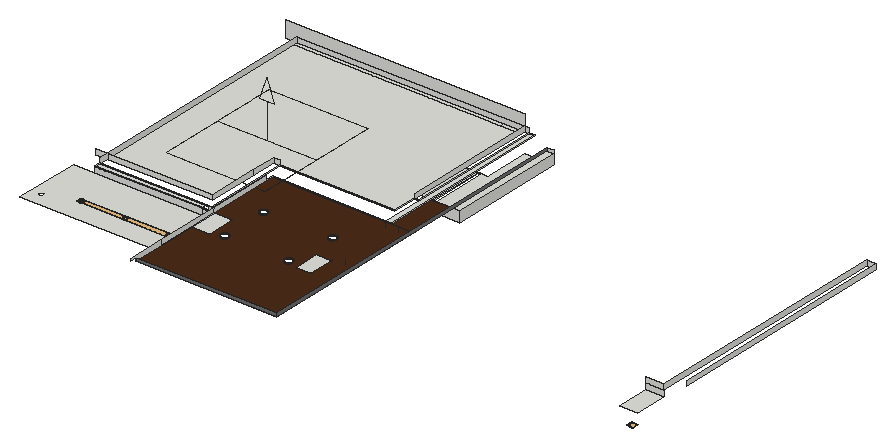
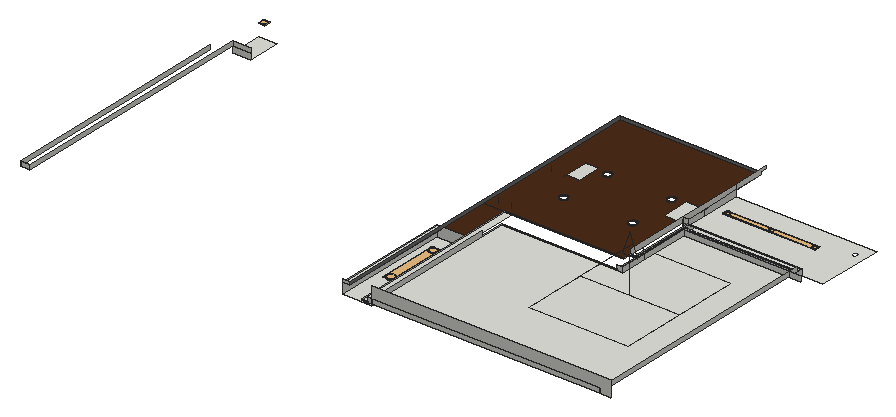
# SketchUp Ruby script. Lengths in inches.
U = 1.inch
M = Sketchup.active_model
def pt(a) = Geom::Point3d.new(a.map { |v| v * U })
def face(e, loops, mat)
  f = e.add_face(loops[0].map { |a| pt(a) })
  loops[1..].each { |l| e.add_face(l.map { |a| pt(a) }).erase! }
  f.material = f.back_material = mat if mat
  f
end
# faces: each face lists its corners as indices into pts; further lists are holes
def faces(e, pts, list, mat = nil) = list.each { |f| face(e, (f[0].is_a?(Array) ? f : [f]).map { |l| l.map { |i| pts[i] } }, mat) }
# xy, xz, yz: faces in a plane at the given z, y or x. An outline is a flat list of corners, or four numbers for a rectangle; further outlines are holes
def ring(l) = l.size == 4 ? [[l[0], l[1]], [l[2], l[1]], [l[2], l[3]], [l[0], l[3]]] : l.each_slice(2).to_a
def flat(e, list, mat, &to3) = list.each { |f| face(e, (f[0].is_a?(Array) ? f : [f]).map { |l| ring(l).map { |u, v| to3.(u, v) } }, mat) }
def xy(e, z, list, mat = nil) = flat(e, list, mat) { |x, y| [x, y, z] }
def xz(e, y, list, mat = nil) = flat(e, list, mat) { |x, z| [x, y, z] }
def yz(e, x, list, mat = nil) = flat(e, list, mat) { |y, z| [x, y, z] }
def lines(e, pts, list) = list.each { |a, b| e.add_line(pt(pts[a]), pt(pts[b])) }
# prism: a flat outline (further loops are holes) pulled along v
def prism(e, loops, v, mat = nil)
  f = face(e, loops, mat); d = Geom::Vector3d.new(v.map { |x| x * U })
  f.pushpull(f.normal.samedirection?(d) ? d.length : -d.length)
end
def box(e, o, s, mat = nil) = prism(e, [[o, [o[0] + s[0], o[1], o[2]], [o[0] + s[0], o[1] + s[1], o[2]], [o[0], o[1] + s[1], o[2]]]], [0, 0, s[2]], mat)
def at(x, y, z, deg = 0) = Geom::Transformation.translation(pt([x, y, z])) * Geom::Transformation.rotation(ORIGIN, Z_AXIS, deg.degrees)
def axes(o, x, y, z) = Geom::Transformation.new([*x, 0, *y, 0, *z, 0, *pt(o).to_a, 1])
def part(name) = M.definitions.add(name)
# library, detail: a bought-in or finely detailed component or shape, given as its bounding box
def library(name, o, s) = part(name).tap { |d| box(d.entities, o, s) }
def detail(e, o, s) = box(e.add_group.entities, o, s)
def put(e, d, t, mat = nil) = e.add_instance(d, t).tap { |i| i.material = mat if mat }
def group(e, t, mat = nil) = e.add_group.tap { |g| g.transformation = t; g.material = mat if mat }.entities
root = M.entities
M.materials.add("[Color M05]").color = [114, 114, 114]
M.materials.add("[Wood Veneer 01]").color = [76, 44, 23]
c1 = library("Group\#20",[-0.5,-0.5,-0.1],[139.5,7.875,0.2])
c2 = part("Group266\#1")
p = [[0,0,0],[0,0,-53.16],[-11.52,0,-53.16],[75.01,-97.09,0],[-75.01,-97.09,0],[75.01,97.09,0],
  [75.01,0,0],[-75.01,97.09,0],[11.52,0,-53.16],[-75.01,0,0],[0,0,-86.05]]
lines(c2.entities,p,[[0,1],[1,2],[3,4],[5,6],[7,5],[1,8],[9,0],[0,6],[8,10],[4,9],[6,3],[2,10],
  [9,7]])
c3 = part("Rectangle Light\#1")
put(c3.entities,c2,at(0,0,0))
c4 = library("Group\#22",[-0.5,-0.5,-0.1],[13.19,93.55,0.2])
c5 = library("Group\#26",[-0.5,-0.5,-0.1],[9.125,9.125,0.2])
xy(root,102.625,[[[2456.54,822.54,2456.54,844.85,2447.32,844.85,2447.32,929.47,2456.54,929.47,2456.54,999.35,2500.29,999.35,2500.29,822.54],[2481.48,926.86,2483.06,927.07,2484.53,927.68,2485.79,928.65,2486.76,929.91,2487.37,931.375,2487.57,932.95,2487.37,934.53,2486.76,936,2485.79,937.26,2484.53,938.23,2483.06,938.84,2481.48,939.05,2479.9,938.84,2478.44,938.23,2477.17,937.26,2476.21,936,2475.6,934.53,2475.39,932.95,2475.6,931.375,2476.21,929.91,2477.17,928.65,2478.44,927.68,2479.9,927.07],[2481.48,846.49,2483.03,846.7,2484.48,847.3,2485.72,848.25,2486.68,849.49,2487.28,850.94,2487.48,852.49,2487.28,854.05,2486.68,855.49,2485.72,856.74,2484.48,857.69,2483.03,858.29,2481.48,858.49,2479.93,858.29,2478.48,857.69,2477.24,856.74,2476.29,855.49,2475.6875,854.05,2475.48,852.49,2475.6875,850.94,2476.29,849.49,2477.24,848.25,2478.48,847.3,2479.93,846.7]],[2348.36,844.85,2442.07,928.79],[2442.07,844.85,2442.76,929.47],[2348.36,928.79,2442.07,929.47],[2442.76,928.79,2443.44,928.79,2443.44,928.91,2447.32,928.91,2447.32,929.47,2442.76,929.47],
  [2443.44,928.79,2447.32,928.91]])
xy(root,109.5,[[2930.51,586.4375,2957.51,636.6875]])
xy(root,109.625,[[[2064.92,536.1875,2276.89,636.6875],[2079.48,553.83,2080.53,553.97,2081.51,554.38,2082.36,555.02,2083,555.87,2083.41,556.85,2083.55,557.9,2083.41,558.95,2083,559.93,2082.36,560.77,2081.51,561.42,2080.53,561.82,2079.48,561.96,2078.43,561.82,2077.45,561.42,2076.61,560.77,2075.96,559.93,2075.56,558.95,2075.42,557.9,2075.56,556.85,2075.96,555.87,2076.61,555.02,2077.45,554.38,2078.43,553.97],[2127.54,570.51,2128.43,570.63,2129.26,570.97,2129.97,571.52,2130.52,572.23,2130.86,573.0625,2130.98,573.95,2130.86,574.84,2130.52,575.67,2129.97,576.38,2129.26,576.93,2128.43,577.27,2127.54,577.39,2126.65,577.27,2125.82,576.93,2125.11,576.38,2124.5625,575.67,2124.22,574.84,2124.1,573.95,2124.22,573.0625,2124.5625,572.23,2125.11,571.52,2125.82,570.97,2126.65,570.63],[2193.35,570.51,2194.24,570.63,2195.07,570.97,2195.78,571.52,2196.33,572.23,2196.67,573.0625,2196.79,573.95,2196.67,574.84,2196.33,575.67,2195.78,576.38,2195.07,576.93,2194.24,577.27,2193.35,577.39,2192.46,577.27,2191.63,576.93,2190.92,576.38,2190.375,575.67,2190.03,574.84,2189.91,573.95,2190.03,573.0625,2190.375,572.23,2190.92,571.52,2191.63,570.97,2192.46,570.63],[2259.16,570.51,2260.05,570.63,2260.88,570.97,2261.6,571.52,2262.14,572.23,2262.48,573.0625,2262.6,573.95,2262.48,574.84,2262.14,575.67,2261.6,576.38,2260.88,576.93,2260.05,577.27,2259.16,577.39,2258.27,577.27,2257.45,576.93,2256.73,576.38,2256.1875,575.67,2255.84,574.84,2255.73,573.95,2255.84,573.0625,2256.1875,572.23,2256.73,571.52,2257.45,570.97,2258.27,570.63]]])
xy(root,118.5,[[2276.89,595.6875,2304.32,636.625],[2435.04,595.6875,2456.54,633.25],[2097.23,636.6875,2258.0625,645.91],[2097.23,660.21,2097.23,1011.63,2440.84,1011.63,2440.84,774.3125,2256.86,774.3125,2256.86,660.21],[2447.32,747.5625,2456.54,1019],
  [2489.98,822.54,2500.29,999.35],[2097.23,1011.63,2409.98,1019],[2409.98,1011.63,2440.84,1019]])
xy(root,118.5,[[[2276.89,488.8125,2276.89,595.6875,2304.32,595.6875,2304.32,636.625,2276.89,636.625,2276.89,747.5625,2489.98,747.5625,2489.98,488.8125],[2435.04,595.6875,2456.54,633.25],[2418.52,595.88,2420.07,596.09,2421.52,596.69,2422.76,597.64,2423.72,598.88,2424.32,600.33,2424.52,601.88,2424.32,603.43,2423.72,604.88,2422.76,606.125,2421.52,607.08,2420.07,607.68,2418.52,607.88,2416.97,607.68,2415.52,607.08,2414.28,606.125,2413.33,604.88,2412.73,603.43,2412.52,601.88,2412.73,600.33,2413.33,598.88,2414.28,597.64,2415.52,596.69,2416.97,596.09],[2424.07,671.87,2425.625,672.07,2427.07,672.67,2428.3125,673.625,2429.27,674.87,2429.87,676.3125,2430.07,677.87,2429.87,679.42,2429.27,680.87,2428.3125,682.11,2427.07,683.0625,2425.625,683.66,2424.07,683.87,2422.52,683.66,2421.07,683.0625,2419.83,682.11,2418.875,680.87,2418.28,679.42,2418.07,677.87,2418.28,676.3125,2418.875,674.87,2419.83,673.625,2421.07,672.67,2422.52,672.07],[2321.71,668.63,2323.26,668.84,2324.71,669.44,2325.95,670.39,2326.91,671.63,2327.5,673.08,2327.71,674.63,2327.5,676.18,2326.91,677.63,2325.95,678.875,2324.71,679.83,2323.26,680.43,2321.71,680.63,2320.16,680.43,2318.71,679.83,2317.47,678.875,2316.51,677.63,2315.91,676.18,2315.71,674.63,2315.91,673.08,2316.51,671.63,2317.47,670.39,2318.71,669.44,2320.16,668.84],[2321.71,595.88,2323.26,596.09,2324.71,596.69,2325.95,597.64,2326.91,598.88,2327.5,600.33,2327.71,601.88,2327.5,603.43,2326.91,604.88,2325.95,606.125,2324.71,607.08,2323.26,607.68,2321.71,607.88,2320.16,607.68,2318.71,607.08,2317.47,606.125,2316.51,604.88,2315.91,603.43,2315.71,601.88,2315.91,600.33,2316.51,598.88,2317.47,597.64,2318.71,596.69,2320.16,596.09]],[2456.54,747.5625,2489.98,822.54]],"[Wood Veneer 01]")
xz(root,488.8125,[[2276.89,118.5,2489.98,122.875]],"[Color M05]")
xz(root,636.6875,[[2930.51,109.5,2957.51,118.5],[2097.23,109.625,2258.0625,118.5],[2258.0625,109.625,2276.89,118.5],[2097.23,118.5,2269.48,119.75],[2269.48,118.5,2276.89,126],
  [2930.51,118.5,2957.51,126]])
xz(root,645.91,[[2097.23,118.5,2266.54,119.75]])
xz(root,660.21,[[2079.65,118.5,2256.86,126]])
xz(root,735.75,[[2269.48,118.5,2276.89,119.75]])
xz(root,747.5625,[[2276.89,118.5,2447.32,119.75],[2447.32,118.5,2456.54,119.75]])
xz(root,774.3125,[[2256.86,118.5,2266.54,126],[2266.54,118.5,2440.84,119.75]])
xz(root,811.54,[[2440.84,118.5,2447.32,119.75]])
xz(root,822.54,[[2456.54,102.625,2500.29,118.5]])
xz(root,999.35,[[2489.98,118.5,2500.29,122.875]])
xz(root,1019,[[2079.65,118.5,2079.65,142.875,2440.84,142.875,2440.84,126,2097.23,126,2097.23,118.5],[2097.23,118.5,2440.84,126],[2440.84,118.5,2447.32,126],[2447.32,118.5,2456.54,119.75],[2957.51,118.5,2972.24,126]])
yz(root,2097.23,[[636.6875,118.5,645.91,119.75],[645.91,118.5,1019,126]])
yz(root,2256.86,[[660.21,118.5,735.75,126],[735.75,118.5,774.3125,126]])
yz(root,2266.54,[[645.91,118.5,774.3125,119.75]])
yz(root,2269.48,[[636.6875,118.5,735.75,119.75]])
yz(root,2276.89,[[536.1875,109.625,595.6875,118.5],[595.6875,109.625,636.625,118.5],[636.625,109.625,636.6875,118.5],[488.8125,118.5,488.8125,122.875,479.5,122.875,479.5,126,536.1875,126,536.1875,118.5],[536.1875,118.5,636.6875,126],
  [636.6875,118.5,735.75,126],[735.75,118.5,747.5625,119.75]])
yz(root,2440.84,[[774.3125,118.5,811.54,119.75],[811.54,118.5,1019,126]])
yz(root,2447.32,[[811.54,118.5,1019,119.75]])
yz(root,2456.54,[[747.5625,118.5,1019,119.75]])
yz(root,2489.98,[[488.8125,118.5,999.35,122.875]],"[Color M05]")
yz(root,2500.29,[[822.54,102.625,999.35,118.5]])
yz(root,2957.51,[[636.6875,118.5,1019,126]])
yz(root,2972.24,[[660.21,118.5,1019,126]])
p = [[2481.48,846.49,102.625],[2479.93,846.7,102.625],[2479.93,846.7,103.9375],[2481.48,846.49,103.9375],[2483.03,846.7,102.625],[2483.03,846.7,103.9375],
  [2478.48,847.3,102.625],[2478.48,847.3,103.9375],[2484.48,847.3,102.625],[2484.48,847.3,103.9375],[2477.24,848.25,102.625],[2477.24,848.25,103.9375],
  [2485.72,848.25,102.625],[2485.72,848.25,103.9375],[2476.29,849.49,102.625],[2476.29,849.49,103.9375],[2486.68,849.49,102.625],[2486.68,849.49,103.9375],
  [2475.6875,850.94,102.625],[2475.6875,850.94,103.9375],[2487.28,850.94,102.625],[2487.28,850.94,103.9375],[2475.48,852.49,102.625],[2475.48,852.49,103.9375],
  [2487.48,852.49,102.625],[2487.48,852.49,103.9375],[2475.6875,854.05,102.625],[2475.6875,854.05,103.9375],[2487.28,854.05,102.625],[2487.28,854.05,103.9375],
  [2476.29,855.49,102.625],[2476.29,855.49,103.9375],[2486.68,855.49,102.625],[2486.68,855.49,103.9375],[2477.24,856.74,102.625],[2477.24,856.74,103.9375],
  [2485.72,856.74,102.625],[2485.72,856.74,103.9375],[2478.48,857.69,102.625],[2478.48,857.69,103.9375],[2484.48,857.69,102.625],[2484.48,857.69,103.9375],
  [2479.93,858.29,102.625],[2479.93,858.29,103.9375],[2483.03,858.29,102.625],[2483.03,858.29,103.9375],[2481.48,858.49,102.625],[2481.48,858.49,103.9375],
  [2481.48,926.86,102.625],[2479.9,927.07,102.625],[2479.9,927.07,103.9375],[2481.48,926.86,103.9375],[2483.06,927.07,102.625],[2483.06,927.07,103.9375],
  [2478.44,927.68,102.625],[2478.44,927.68,103.9375],[2484.53,927.68,102.625],[2484.53,927.68,103.9375],[2477.17,928.65,102.625],[2477.17,928.65,103.9375],
  [2485.79,928.65,102.625],[2485.79,928.65,103.9375],[2476.21,929.91,102.625],[2476.21,929.91,103.9375],[2486.76,929.91,102.625],[2486.76,929.91,103.9375],
  [2475.6,931.375,102.625],[2475.6,931.375,103.9375],[2487.37,931.375,102.625],[2487.37,931.375,103.9375],[2475.39,932.95,102.625],[2475.39,932.95,103.9375],
  [2487.57,932.95,102.625],[2487.57,932.95,103.9375],[2475.6,934.53,102.625],[2475.6,934.53,103.9375],[2487.37,934.53,102.625],[2487.37,934.53,103.9375],
  [2476.21,936,102.625],[2476.21,936,103.9375],[2486.76,936,102.625],[2486.76,936,103.9375],[2477.17,937.26,102.625],[2477.17,937.26,103.9375],
  [2485.79,937.26,102.625],[2485.79,937.26,103.9375],[2478.44,938.23,102.625],[2478.44,938.23,103.9375],[2484.53,938.23,102.625],[2484.53,938.23,103.9375],
  [2479.9,938.84,102.625],[2479.9,938.84,103.9375],[2483.06,938.84,102.625],[2483.06,938.84,103.9375],[2481.48,939.05,102.625],[2481.48,939.05,103.9375],
  [2972.07,553.83,109.625],[2971.02,553.97,109.625],[2971.02,553.97,110.5625],[2972.07,553.83,110.5625],[2970.04,554.38,109.625],[2970.04,554.38,110.5625],
  [2969.2,555.02,109.625],[2969.2,555.02,110.5625],[2968.55,555.87,109.625],[2968.55,555.87,110.5625],[2968.15,556.85,109.625],[2968.15,556.85,110.5625],
  [2968.01,557.9,109.625],[2968.01,557.9,110.5625],[2968.15,558.95,109.625],[2968.15,558.95,110.5625],[2968.55,559.93,109.625],[2968.55,559.93,110.5625],
  [2969.2,560.77,109.625],[2969.2,560.77,110.5625],[2970.04,561.42,109.625],[2970.04,561.42,110.5625],[2971.02,561.82,109.625],[2971.02,561.82,110.5625],
  [2972.07,561.96,109.625],[2972.07,561.96,110.5625],[2127.54,570.51,109.625],[2126.65,570.63,109.625],[2126.65,570.63,110.0625],[2127.54,570.51,110.0625],
  [2128.43,570.63,109.625],[2128.43,570.63,110.0625],[2193.35,570.51,109.625],[2192.46,570.63,109.625],[2192.46,570.63,110.0625],[2193.35,570.51,110.0625],
  [2194.24,570.63,109.625],[2194.24,570.63,110.0625],[2259.16,570.51,109.625],[2258.27,570.63,109.625],[2258.27,570.63,110.0625],[2259.16,570.51,110.0625],
  [2260.05,570.63,109.625],[2260.05,570.63,110.0625],[2125.82,570.97,109.625],[2125.82,570.97,110.0625],[2129.26,570.97,109.625],[2129.26,570.97,110.0625],
  [2191.63,570.97,109.625],[2191.63,570.97,110.0625],[2195.07,570.97,109.625],[2195.07,570.97,110.0625],[2257.45,570.97,109.625],[2257.45,570.97,110.0625],
  [2260.88,570.97,109.625],[2260.88,570.97,110.0625],[2125.11,571.52,109.625],[2125.11,571.52,110.0625],[2129.97,571.52,109.625],[2129.97,571.52,110.0625],
  [2190.92,571.52,109.625],[2190.92,571.52,110.0625],[2195.78,571.52,109.625],[2195.78,571.52,110.0625],[2256.73,571.52,109.625],[2256.73,571.52,110.0625],
  [2261.6,571.52,109.625],[2261.6,571.52,110.0625],[2124.5625,572.23,109.625],[2124.5625,572.23,110.0625],[2130.52,572.23,109.625],[2130.52,572.23,110.0625],
  [2190.375,572.23,109.625],[2190.375,572.23,110.0625],[2196.33,572.23,109.625],[2196.33,572.23,110.0625],[2256.1875,572.23,109.625],[2256.1875,572.23,110.0625],
  [2262.14,572.23,109.625],[2262.14,572.23,110.0625],[2124.22,573.0625,109.625],[2124.22,573.0625,110.0625],[2130.86,573.0625,109.625],[2130.86,573.0625,110.0625],
  [2190.03,573.0625,109.625],[2190.03,573.0625,110.0625],[2196.67,573.0625,109.625],[2196.67,573.0625,110.0625],[2255.84,573.0625,109.625],[2255.84,573.0625,110.0625],
  [2262.48,573.0625,109.625],[2262.48,573.0625,110.0625],[2124.1,573.95,109.625],[2124.1,573.95,110.0625],[2130.98,573.95,109.625],[2130.98,573.95,110.0625],
  [2189.91,573.95,109.625],[2189.91,573.95,110.0625],[2196.79,573.95,109.625],[2196.79,573.95,110.0625],[2255.73,573.95,109.625],[2255.73,573.95,110.0625],
  [2262.6,573.95,109.625],[2262.6,573.95,110.0625],[2124.22,574.84,109.625],[2124.22,574.84,110.0625],[2130.86,574.84,109.625],[2130.86,574.84,110.0625],
  [2190.03,574.84,109.625],[2190.03,574.84,110.0625],[2196.67,574.84,109.625],[2196.67,574.84,110.0625],[2255.84,574.84,109.625],[2255.84,574.84,110.0625],
  [2262.48,574.84,109.625],[2262.48,574.84,110.0625],[2124.5625,575.67,109.625],[2124.5625,575.67,110.0625],[2130.52,575.67,109.625],[2130.52,575.67,110.0625],
  [2190.375,575.67,109.625],[2190.375,575.67,110.0625],[2196.33,575.67,109.625],[2196.33,575.67,110.0625],[2256.1875,575.67,109.625],[2256.1875,575.67,110.0625],
  [2262.14,575.67,109.625],[2262.14,575.67,110.0625],[2125.11,576.38,109.625],[2125.11,576.38,110.0625],[2129.97,576.38,109.625],[2129.97,576.38,110.0625],
  [2190.92,576.38,109.625],[2190.92,576.38,110.0625],[2195.78,576.38,109.625],[2195.78,576.38,110.0625],[2256.73,576.38,109.625],[2256.73,576.38,110.0625],
  [2261.6,576.38,109.625],[2261.6,576.38,110.0625],[2125.82,576.93,109.625],[2125.82,576.93,110.0625],[2129.26,576.93,109.625],[2129.26,576.93,110.0625],
  [2191.63,576.93,109.625],[2191.63,576.93,110.0625],[2195.07,576.93,109.625],[2195.07,576.93,110.0625],[2257.45,576.93,109.625],[2257.45,576.93,110.0625],
  [2260.88,576.93,109.625],[2260.88,576.93,110.0625],[2126.65,577.27,109.625],[2126.65,577.27,110.0625],[2128.43,577.27,109.625],[2128.43,577.27,110.0625],
  [2192.46,577.27,109.625],[2192.46,577.27,110.0625],[2194.24,577.27,109.625],[2194.24,577.27,110.0625],[2258.27,577.27,109.625],[2258.27,577.27,110.0625],
  [2260.05,577.27,109.625],[2260.05,577.27,110.0625],[2127.54,577.39,109.625],[2127.54,577.39,110.0625],[2193.35,577.39,109.625],[2193.35,577.39,110.0625],
  [2259.16,577.39,109.625],[2259.16,577.39,110.0625],[2321.71,595.88,118.5],[2320.16,596.09,118.5],[2320.16,596.09,119.375],[2321.71,595.88,119.375],
  [2323.26,596.09,118.5],[2323.26,596.09,119.375],[2418.52,595.88,118.5],[2416.97,596.09,118.5],[2416.97,596.09,119.375],[2418.52,595.88,119.375],
  [2420.07,596.09,118.5],[2420.07,596.09,119.375],[2318.71,596.69,118.5],[2318.71,596.69,119.375],[2324.71,596.69,118.5],[2324.71,596.69,119.375],
  [2415.52,596.69,118.5],[2415.52,596.69,119.375],[2421.52,596.69,118.5],[2421.52,596.69,119.375],[2317.47,597.64,118.5],[2317.47,597.64,119.375],
  [2325.95,597.64,118.5],[2325.95,597.64,119.375],[2414.28,597.64,118.5],[2414.28,597.64,119.375],[2422.76,597.64,118.5],[2422.76,597.64,119.375],
  [2316.51,598.88,118.5],[2316.51,598.88,119.375],[2326.91,598.88,118.5],[2326.91,598.88,119.375],[2413.33,598.88,118.5],[2413.33,598.88,119.375],
  [2423.72,598.88,118.5],[2423.72,598.88,119.375],[2315.91,600.33,118.5],[2315.91,600.33,119.375],[2327.5,600.33,118.5],[2327.5,600.33,119.375],
  [2412.73,600.33,118.5],[2412.73,600.33,119.375],[2424.32,600.33,118.5],[2424.32,600.33,119.375],[2315.71,601.88,118.5],[2315.71,601.88,119.375],
  [2327.71,601.88,118.5],[2327.71,601.88,119.375],[2412.52,601.88,118.5],[2412.52,601.88,119.375],[2424.52,601.88,118.5],[2424.52,601.88,119.375],
  [2315.91,603.43,118.5],[2315.91,603.43,119.375],[2327.5,603.43,118.5],[2327.5,603.43,119.375],[2412.73,603.43,118.5],[2412.73,603.43,119.375],
  [2424.32,603.43,118.5],[2424.32,603.43,119.375],[2316.51,604.88,118.5],[2316.51,604.88,119.375],[2326.91,604.88,118.5],[2326.91,604.88,119.375],
  [2413.33,604.88,118.5],[2413.33,604.88,119.375],[2423.72,604.88,118.5],[2423.72,604.88,119.375],[2317.47,606.125,118.5],[2317.47,606.125,119.375],
  [2325.95,606.125,118.5],[2325.95,606.125,119.375],[2414.28,606.125,118.5],[2414.28,606.125,119.375],[2422.76,606.125,118.5],[2422.76,606.125,119.375],
  [2318.71,607.08,118.5],[2318.71,607.08,119.375],[2324.71,607.08,118.5],[2324.71,607.08,119.375],[2415.52,607.08,118.5],[2415.52,607.08,119.375],
  [2421.52,607.08,118.5],[2421.52,607.08,119.375],[2320.16,607.68,118.5],[2320.16,607.68,119.375],[2323.26,607.68,118.5],[2323.26,607.68,119.375],
  [2416.97,607.68,118.5],[2416.97,607.68,119.375],[2420.07,607.68,118.5],[2420.07,607.68,119.375],[2321.71,607.88,118.5],[2321.71,607.88,119.375],
  [2418.52,607.88,118.5],[2418.52,607.88,119.375],[2321.71,668.63,118.5],[2320.16,668.84,118.5],[2320.16,668.84,119.375],[2321.71,668.63,119.375],
  [2323.26,668.84,118.5],[2323.26,668.84,119.375],[2318.71,669.44,118.5],[2318.71,669.44,119.375],[2324.71,669.44,118.5],[2324.71,669.44,119.375],
  [2317.47,670.39,118.5],[2317.47,670.39,119.375],[2325.95,670.39,118.5],[2325.95,670.39,119.375],[2316.51,671.63,118.5],[2316.51,671.63,119.375],
  [2326.91,671.63,118.5],[2326.91,671.63,119.375],[2315.91,673.08,118.5],[2315.91,673.08,119.375],[2327.5,673.08,118.5],[2327.5,673.08,119.375],
  [2424.07,671.87,118.5],[2422.52,672.07,118.5],[2422.52,672.07,119.375],[2424.07,671.87,119.375],[2425.625,672.07,118.5],[2425.625,672.07,119.375],
  [2421.07,672.67,118.5],[2421.07,672.67,119.375],[2427.07,672.67,118.5],[2427.07,672.67,119.375],[2419.83,673.625,118.5],[2419.83,673.625,119.375],
  [2428.3125,673.625,118.5],[2428.3125,673.625,119.375],[2315.71,674.63,118.5],[2315.71,674.63,119.375],[2327.71,674.63,118.5],[2327.71,674.63,119.375],
  [2418.875,674.87,118.5],[2418.875,674.87,119.375],[2429.27,674.87,118.5],[2429.27,674.87,119.375],[2315.91,676.18,118.5],[2315.91,676.18,119.375],
  [2327.5,676.18,118.5],[2327.5,676.18,119.375],[2418.28,676.3125,118.5],[2418.28,676.3125,119.375],[2429.87,676.3125,118.5],[2429.87,676.3125,119.375],
  [2316.51,677.63,118.5],[2316.51,677.63,119.375],[2326.91,677.63,118.5],[2326.91,677.63,119.375],[2418.07,677.87,118.5],[2418.07,677.87,119.375],
  [2430.07,677.87,118.5],[2430.07,677.87,119.375],[2317.47,678.875,118.5],[2317.47,678.875,119.375],[2325.95,678.875,118.5],[2325.95,678.875,119.375],
  [2418.28,679.42,118.5],[2418.28,679.42,119.375],[2429.87,679.42,118.5],[2429.87,679.42,119.375],[2318.71,679.83,118.5],[2318.71,679.83,119.375],
  [2324.71,679.83,118.5],[2324.71,679.83,119.375],[2418.875,680.87,118.5],[2418.875,680.87,119.375],[2429.27,680.87,118.5],[2429.27,680.87,119.375],
  [2320.16,680.43,118.5],[2320.16,680.43,119.375],[2323.26,680.43,118.5],[2323.26,680.43,119.375],[2321.71,680.63,118.5],[2321.71,680.63,119.375],
  [2419.83,682.11,118.5],[2419.83,682.11,119.375],[2428.3125,682.11,118.5],[2428.3125,682.11,119.375],[2421.07,683.0625,118.5],[2421.07,683.0625,119.375],
  [2427.07,683.0625,118.5],[2427.07,683.0625,119.375],[2422.52,683.66,118.5],[2422.52,683.66,119.375],[2425.625,683.66,118.5],[2425.625,683.66,119.375],
  [2424.07,683.87,118.5],[2424.07,683.87,119.375],[2456.54,735.75,126],[2456.54,735.75,118.5],[2475.98,735.75,126],[2475.98,735.75,118.5],
  [2475.98,636.6875,118.5],[2475.98,636.6875,126],[2475.98,636.625,118.5],[2456.54,636.625,118.5],[2456.54,633.25,118.5]]
faces(root,p,[[0,1,2,3],[4,0,3,5],[1,6,7,2],[8,4,5,9],[6,10,11,7],[12,8,9,13],[10,14,15,11],[16,12,13,17],
  [14,18,19,15],[20,16,17,21],[18,22,23,19],[24,20,21,25],[22,26,27,23],[28,24,25,29],[26,30,31,27],[32,28,29,33],
  [30,34,35,31],[36,32,33,37],[34,38,39,35],[40,36,37,41],[38,42,43,39],[44,40,41,45],[42,46,47,43],[46,44,45,47],
  [48,49,50,51],[52,48,51,53],[49,54,55,50],[56,52,53,57],[54,58,59,55],[60,56,57,61],[58,62,63,59],[64,60,61,65],
  [62,66,67,63],[68,64,65,69],[66,70,71,67],[72,68,69,73],[70,74,75,71],[76,72,73,77],[74,78,79,75],[80,76,77,81],
  [78,82,83,79],[84,80,81,85],[82,86,87,83],[88,84,85,89],[86,90,91,87],[92,88,89,93],[90,94,95,91],[94,92,93,95],
  [96,97,98,99],[97,100,101,98],[100,102,103,101],[102,104,105,103],[104,106,107,105],[106,108,109,107],[108,110,111,109],[110,112,113,111],
  [112,114,115,113],[114,116,117,115],[116,118,119,117],[118,120,121,119],[122,123,124,125],[126,122,125,127],[128,129,130,131],[132,128,131,133],
  [134,135,136,137],[138,134,137,139],[123,140,141,124],[142,126,127,143],[129,144,145,130],[146,132,133,147],[135,148,149,136],[150,138,139,151],
  [140,152,153,141],[154,142,143,155],[144,156,157,145],[158,146,147,159],[148,160,161,149],[162,150,151,163],[152,164,165,153],[166,154,155,167],
  [156,168,169,157],[170,158,159,171],[160,172,173,161],[174,162,163,175],[164,176,177,165],[178,166,167,179],[168,180,181,169],[182,170,171,183],
  [172,184,185,173],[186,174,175,187],[176,188,189,177],[190,178,179,191],[180,192,193,181],[194,182,183,195],[184,196,197,185],[198,186,187,199],
  [188,200,201,189],[202,190,191,203],[192,204,205,193],[206,194,195,207],[196,208,209,197],[210,198,199,211],[200,212,213,201],[214,202,203,215],
  [204,216,217,205],[218,206,207,219],[208,220,221,209],[222,210,211,223],[212,224,225,213],[226,214,215,227],[216,228,229,217],[230,218,219,231],
  [220,232,233,221],[234,222,223,235],[224,236,237,225],[238,226,227,239],[228,240,241,229],[242,230,231,243],[232,244,245,233],[246,234,235,247],
  [236,248,249,237],[250,238,239,251],[240,252,253,241],[254,242,243,255],[244,256,257,245],[258,246,247,259],[248,260,261,249],[260,250,251,261],
  [252,262,263,253],[262,254,255,263],[256,264,265,257],[264,258,259,265]])
faces(root,p,[[266,267,268,269],[270,266,269,271],[272,273,274,275],[276,272,275,277],[267,278,279,268],[280,270,271,281],[273,282,283,274],[284,276,277,285],
  [278,286,287,279],[288,280,281,289],[282,290,291,283],[292,284,285,293],[286,294,295,287],[296,288,289,297],[290,298,299,291],[300,292,293,301],
  [294,302,303,295],[304,296,297,305],[298,306,307,299],[308,300,301,309],[302,310,311,303],[312,304,305,313],[306,314,315,307],[316,308,309,317],
  [310,318,319,311],[320,312,313,321],[314,322,323,315],[324,316,317,325],[318,326,327,319],[328,320,321,329],[322,330,331,323],[332,324,325,333],
  [326,334,335,327],[336,328,329,337],[330,338,339,331],[340,332,333,341],[334,342,343,335],[344,336,337,345],[338,346,347,339],[348,340,341,349],
  [342,350,351,343],[352,344,345,353],[346,354,355,347],[356,348,349,357],[350,358,359,351],[358,352,353,359],[354,360,361,355],[360,356,357,361],
  [362,363,364,365],[366,362,365,367],[363,368,369,364],[370,366,367,371],[368,372,373,369],[374,370,371,375],[372,376,377,373],[378,374,375,379],
  [376,380,381,377],[382,378,379,383],[384,385,386,387],[388,384,387,389],[385,390,391,386],[392,388,389,393],[390,394,395,391],[396,392,393,397],
  [380,398,399,381],[400,382,383,401],[394,402,403,395],[404,396,397,405],[398,406,407,399],[408,400,401,409],[402,410,411,403],[412,404,405,413],
  [406,414,415,407],[416,408,409,417],[410,418,419,411],[420,412,413,421],[414,422,423,415],[424,416,417,425],[418,426,427,419],[428,420,421,429],
  [422,430,431,423],[432,424,425,433],[426,434,435,427],[436,428,429,437],[430,438,439,431],[440,432,433,441],[438,442,443,439],[442,440,441,443],
  [434,444,445,435],[446,436,437,447],[444,448,449,445],[450,446,447,451],[448,452,453,449],[454,450,451,455],[452,456,457,453],[456,454,455,457]],"[Wood Veneer 01]")
lines(root,p,[[458,459],[460,461],[462,463],[462,464],[465,466]])
put(root,c1,at(2124.1,570.51,110.0625))
put(root,c3,axes([2216.51,812.42,118.51],[1,0,0],[0,1,0],[0,0,-1]))
put(root,c4,at(2475.39,846.49,103.9375))
put(root,c5,at(2968.01,553.83,110.5625))
